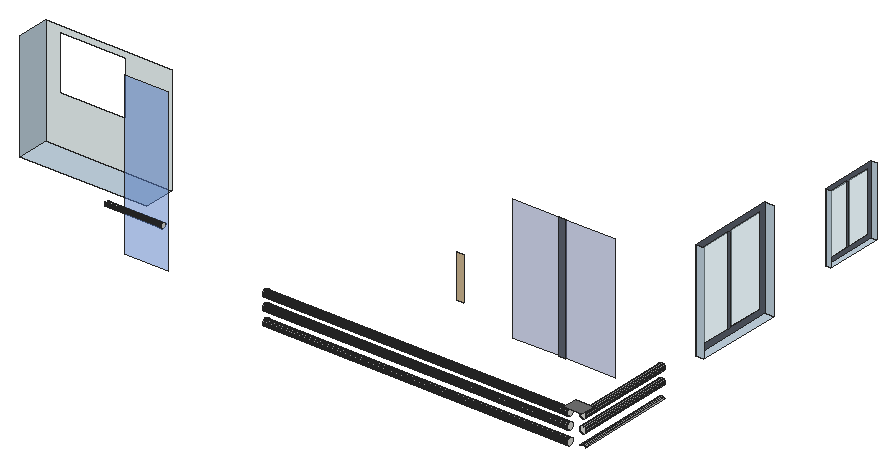
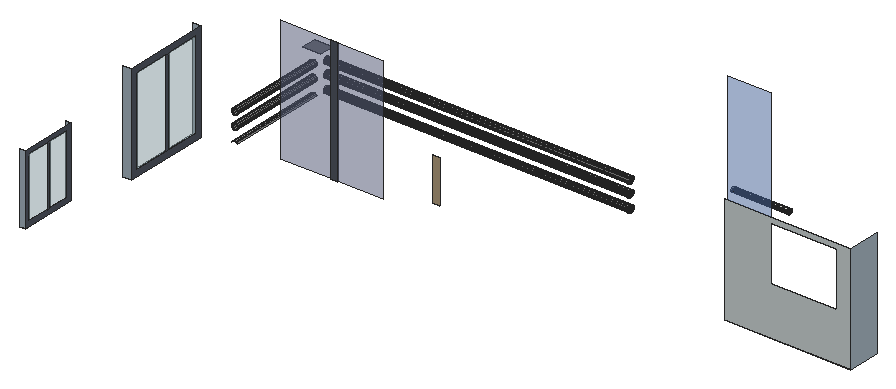
# SketchUp Ruby script. Lengths in inches.
U = 1.inch
M = Sketchup.active_model
def pt(a) = Geom::Point3d.new(a.map { |v| v * U })
def face(e, loops, mat)
  f = e.add_face(loops[0].map { |a| pt(a) })
  loops[1..].each { |l| e.add_face(l.map { |a| pt(a) }).erase! }
  f.material = f.back_material = mat if mat
  f
end
# faces: each face lists its corners as indices into pts; further lists are holes
def faces(e, pts, list, mat = nil) = list.each { |f| face(e, (f[0].is_a?(Array) ? f : [f]).map { |l| l.map { |i| pts[i] } }, mat) }
# xy, xz, yz: faces in a plane at the given z, y or x. An outline is a flat list of corners, or four numbers for a rectangle; further outlines are holes
def ring(l) = l.size == 4 ? [[l[0], l[1]], [l[2], l[1]], [l[2], l[3]], [l[0], l[3]]] : l.each_slice(2).to_a
def flat(e, list, mat, &to3) = list.each { |f| face(e, (f[0].is_a?(Array) ? f : [f]).map { |l| ring(l).map { |u, v| to3.(u, v) } }, mat) }
def xy(e, z, list, mat = nil) = flat(e, list, mat) { |x, y| [x, y, z] }
def xz(e, y, list, mat = nil) = flat(e, list, mat) { |x, z| [x, y, z] }
def yz(e, x, list, mat = nil) = flat(e, list, mat) { |y, z| [x, y, z] }
def lines(e, pts, list) = list.each { |a, b| e.add_line(pt(pts[a]), pt(pts[b])) }
# prism: a flat outline (further loops are holes) pulled along v
def prism(e, loops, v, mat = nil)
  f = face(e, loops, mat); d = Geom::Vector3d.new(v.map { |x| x * U })
  f.pushpull(f.normal.samedirection?(d) ? d.length : -d.length)
end
def box(e, o, s, mat = nil) = prism(e, [[o, [o[0] + s[0], o[1], o[2]], [o[0] + s[0], o[1] + s[1], o[2]], [o[0], o[1] + s[1], o[2]]]], [0, 0, s[2]], mat)
def at(x, y, z, deg = 0) = Geom::Transformation.translation(pt([x, y, z])) * Geom::Transformation.rotation(ORIGIN, Z_AXIS, deg.degrees)
def axes(o, x, y, z) = Geom::Transformation.new([*x, 0, *y, 0, *z, 0, *pt(o).to_a, 1])
def part(name) = M.definitions.add(name)
# library, detail: a bought-in or finely detailed component or shape, given as its bounding box
def library(name, o, s) = part(name).tap { |d| box(d.entities, o, s) }
def detail(e, o, s) = box(e.add_group.entities, o, s)
def put(e, d, t, mat = nil) = e.add_instance(d, t).tap { |i| i.material = mat if mat }
def group(e, t, mat = nil) = e.add_group.tap { |g| g.transformation = t; g.material = mat if mat }.entities
root = M.entities
M.materials.add("[Color M03]").color = [170, 170, 170]
M.materials.add("[Color M05]").color = [114, 114, 114]
M.materials.add("[Formica Beige]").color = [211, 187, 149]
M.materials.add("[Formica Laminate Dark]").color = [95, 101, 114]
M.materials.add("[Terrazzo Light Blue]1").color = [196, 214, 227]
M.materials.add("[Translucent Glass Blue]").color = [100, 149, 237]
M.materials["[Translucent Glass Blue]"].alpha = 0.5
M.materials.add("[Translucent Glass Safety]").color = [204, 235, 244]
M.materials["[Translucent Glass Safety]"].alpha = 0.5
M.materials.add("[Translucent Glass Sky Reflection]").color = [126, 138, 183]
M.materials["[Translucent Glass Sky Reflection]"].alpha = 0.52
M.materials.add("[White Subway Tile]").color = [243, 252, 253]
xy(root,1272.1,[[547.35,1118.14,1034.97,1239.01]],"[Terrazzo Light Blue]1")
xy(root,1302.22,[[2936.43,1390.76,2968.68,1726.13]],"[Terrazzo Light Blue]1")
xy(root,1339.25,[[2140.61,820.84,2143.62,821.24,2146.42,822.4,2148.83,824.25,2150.67,826.66,2151.84,829.46,2152.23,832.47,2151.84,835.48,2150.67,838.28,2148.83,840.69,2146.42,842.54,2143.62,843.7,2140.61,844.09,2137.6,843.7,2134.79,842.54,2132.39,840.69,2130.54,838.28,2129.38,835.48,2128.98,832.47,2129.38,829.46,2130.54,826.66,2132.39,824.25,2134.79,822.4,2137.6,821.24]])
xy(root,1348.11,[[2949.18,2002.64,2968.68,2223.02]],"[Terrazzo Light Blue]1")
xy(root,1369.75,[[2898.76,803.71,2968.68,859.31]],"[Color M05]")
xy(root,1433.45,[[1250.58,820.58,1251.73,820.73,1252.8,821.17,1253.72,821.88,1254.42,822.8,1254.87,823.87,1255.02,825.02,1254.87,826.17,1254.42,827.24,1253.72,828.15,1252.8,828.86,1251.73,829.3,1250.58,829.45,1249.43,829.3,1248.36,828.86,1247.44,828.15,1246.74,827.24,1246.29,826.17,1246.14,825.02,1246.29,823.87,1246.74,822.8,1247.44,821.88,1248.36,821.17,1249.43,820.73]])
xy(root,1436.77,[[1314.2,820.58,1315.35,820.73,1316.42,821.17,1317.34,821.88,1318.05,822.8,1318.49,823.87,1318.64,825.02,1318.49,826.17,1318.05,827.24,1317.34,828.15,1316.42,828.86,1315.35,829.3,1314.2,829.45,1313.06,829.3,1311.99,828.86,1311.07,828.15,1310.36,827.24,1309.92,826.17,1309.77,825.02,1309.92,823.87,1310.36,822.8,1311.07,821.88,1311.99,821.17,1313.06,820.73]])
xy(root,1437.08,[[1197.58,820.58,1198.73,820.73,1199.8,821.17,1200.72,821.88,1201.42,822.8,1201.87,823.87,1202.02,825.02,1201.87,826.17,1201.42,827.24,1200.72,828.15,1199.8,828.86,1198.73,829.3,1197.58,829.45,1196.43,829.3,1195.36,828.86,1194.44,828.15,1193.74,827.24,1193.29,826.17,1193.14,825.02,1193.29,823.87,1193.74,822.8,1194.44,821.88,1195.36,821.17,1196.43,820.73]])
xy(root,1437.8,[[1292.95,820.58,1294.1,820.73,1295.17,821.17,1296.09,821.88,1296.8,822.8,1297.24,823.87,1297.39,825.02,1297.24,826.17,1296.8,827.24,1296.09,828.15,1295.17,828.86,1294.1,829.3,1292.95,829.45,1291.81,829.3,1290.74,828.86,1289.82,828.15,1289.11,827.24,1288.67,826.17,1288.52,825.02,1288.67,823.87,1289.11,822.8,1289.82,821.88,1290.74,821.17,1291.81,820.73]])
xy(root,1440.11,[[1222.58,820.58,1223.73,820.73,1224.8,821.17,1225.72,821.88,1226.42,822.8,1226.87,823.87,1227.02,825.02,1226.87,826.17,1226.42,827.24,1225.72,828.15,1224.8,828.86,1223.73,829.3,1222.58,829.45,1221.43,829.3,1220.36,828.86,1219.44,828.15,1218.74,827.24,1218.29,826.17,1218.14,825.02,1218.29,823.87,1218.74,822.8,1219.44,821.88,1220.36,821.17,1221.43,820.73],[1271.08,820.58,1272.23,820.73,1273.3,821.17,1274.22,821.88,1274.92,822.8,1275.37,823.87,1275.52,825.02,1275.37,826.17,1274.92,827.24,1274.22,828.15,1273.3,828.86,1272.23,829.3,1271.08,829.45,1269.93,829.3,1268.86,828.86,1267.94,828.15,1267.24,827.24,1266.79,826.17,1266.64,825.02,1266.79,823.87,1267.24,822.8,1267.94,821.88,1268.86,821.17,1269.93,820.73]])
xy(root,1442.27,[[1131.58,820.58,1132.73,820.73,1133.8,821.17,1134.72,821.88,1135.42,822.8,1135.87,823.87,1136.02,825.02,1135.87,826.17,1135.42,827.24,1134.72,828.15,1133.8,828.86,1132.73,829.3,1131.58,829.45,1130.43,829.3,1129.36,828.86,1128.44,828.15,1127.74,827.24,1127.29,826.17,1127.14,825.02,1127.29,823.87,1127.74,822.8,1128.44,821.88,1129.36,821.17,1130.43,820.73],[1151.52,820.58,1152.67,820.73,1153.74,821.17,1154.65,821.88,1155.36,822.8,1155.8,823.87,1155.95,825.02,1155.8,826.17,1155.36,827.24,1154.65,828.15,1153.74,828.86,1152.67,829.3,1151.52,829.45,1150.37,829.3,1149.3,828.86,1148.38,828.15,1147.67,827.24,1147.23,826.17,1147.08,825.02,1147.23,823.87,1147.67,822.8,1148.38,821.88,1149.3,821.17,1150.37,820.73],[1173.58,820.58,1174.73,820.73,1175.8,821.17,1176.72,821.88,1177.42,822.8,1177.87,823.87,1178.02,825.02,1177.87,826.17,1177.42,827.24,1176.72,828.15,1175.8,828.86,1174.73,829.3,1173.58,829.45,1172.43,829.3,1171.36,828.86,1170.44,828.15,1169.74,827.24,1169.29,826.17,1169.14,825.02,1169.29,823.87,1169.74,822.8,1170.44,821.88,1171.36,821.17,1172.43,820.73]])
xz(root,859.31,[[2927.58,1264.46,2930.84,1264.89,2933.87,1266.15,2936.47,1268.14,2938.46,1270.75,2939.72,1273.77,2940.15,1277.03,2939.72,1280.28,2938.46,1283.31,2936.47,1285.91,2933.87,1287.91,2930.84,1289.16,2927.58,1289.59,2924.33,1289.16,2921.3,1287.91,2918.7,1285.91,2916.7,1283.31,2915.45,1280.28,2915.02,1277.03,2915.45,1273.77,2916.7,1270.75,2918.7,1268.14,2921.3,1266.15,2924.33,1264.89],[2927.58,1316.03,2930.84,1316.45,2933.87,1317.71,2936.47,1319.71,2938.46,1322.31,2939.72,1325.34,2940.15,1328.59,2939.72,1331.84,2938.46,1334.87,2936.47,1337.47,2933.87,1339.47,2930.84,1340.72,2927.58,1341.15,2924.33,1340.72,2921.3,1339.47,2918.7,1337.47,2916.7,1334.87,2915.45,1331.84,2915.02,1328.59,2915.45,1325.34,2916.7,1322.31,2918.7,1319.71,2921.3,1317.71,2924.33,1316.45]])
xz(root,884.27,[[1137.95,1242.25,1309.12,1865.04]],"[Translucent Glass Blue]")
xz(root,1239.01,[[2136.34,1281.23,2162.72,1446.98]],"[Formica Beige]")
xz(root,1239.01,[[2528.23,1224.02,2557.29,1706.3]],"[Formica Laminate Dark]")
xz(root,1239.01,[[2353.98,1224.02,2528.23,1706.3],[2557.29,1224.02,2749.1875,1706.3]],"[Translucent Glass Sky Reflection]")
xz(root,1239.01,[[[547.35,1272.1,1034.97,1690.66],[601.67,1457.66,858.23,1670.72]]],"[White Subway Tile]")
xz(root,1390.76,[[2936.43,1302.22,2968.68,1686.6]],"[Terrazzo Light Blue]1")
xz(root,1726.13,[[2936.43,1302.22,2968.68,1686.6]],"[Terrazzo Light Blue]1")
xz(root,2002.64,[[2949.18,1348.11,2968.68,1615.93]],"[Terrazzo Light Blue]1")
xz(root,2223.02,[[2949.18,1348.11,2968.68,1615.93]],"[Terrazzo Light Blue]1")
yz(root,547.35,[[1118.14,1272.1,1239.01,1690.66]],"[Terrazzo Light Blue]1")
yz(root,1334.04,[[826.07,1428.86,828.38,1429.16,830.54,1430.06,832.39,1431.48,833.8125,1433.33,834.7,1435.48,835.01,1437.8,834.7,1440.11,833.8125,1442.27,832.39,1444.12,830.54,1445.54,828.38,1446.43,826.07,1446.73,823.76,1446.43,821.6,1445.54,819.75,1444.12,818.33,1442.27,817.4375,1440.11,817.13,1437.8,817.4375,1435.48,818.33,1433.33,819.75,1431.48,821.6,1430.06,823.76,1429.16]])
yz(root,2898.76,[[834.19,1224.6,837.45,1225.03,840.48,1226.29,843.08,1228.28,845.07,1230.88,846.33,1233.91,846.76,1237.17,846.33,1240.42,845.07,1243.45,843.08,1246.05,840.48,1248.05,837.45,1249.3,834.19,1249.73,830.94,1249.3,827.91,1248.05,825.3125,1246.05,823.32,1243.45,822.06,1240.42,821.63,1237.17,822.06,1233.91,823.32,1230.88,825.3125,1228.28,827.91,1226.29,830.94,1225.03],[834.19,1277.73,837.45,1278.16,840.48,1279.41,843.08,1281.41,845.07,1284.01,846.33,1287.04,846.76,1290.29,846.33,1293.54,845.07,1296.57,843.08,1299.17,840.48,1301.17,837.45,1302.43,834.19,1302.85,830.94,1302.43,827.91,1301.17,825.3125,1299.17,823.32,1296.57,822.06,1293.54,821.63,1290.29,822.06,1287.04,823.32,1284.01,825.3125,1281.41,827.91,1279.41,830.94,1278.16],[834.19,1325.79,837.45,1326.22,840.48,1327.47,843.08,1329.47,845.07,1332.07,846.33,1335.1,846.76,1338.35,846.33,1341.6,845.07,1344.63,843.08,1347.24,840.48,1349.23,837.45,1350.49,834.19,1350.92,830.94,1350.49,827.91,1349.23,825.3125,1347.24,823.32,1344.63,822.06,1341.6,821.63,1338.35,822.06,1335.1,823.32,1332.07,825.3125,1329.47,827.91,1327.47,830.94,1326.22]])
yz(root,2936.43,[[[1390.76,1302.22,1726.13,1686.6],[1414.45,1325.92,1702.4375,1662.9]],[1545.625,1325.92,1562.55,1662.9]],"[Formica Laminate Dark]")
yz(root,2936.43,[[1414.45,1325.92,1545.625,1662.9],[1562.55,1325.92,1702.4375,1662.9]],"[Translucent Glass Safety]")
yz(root,2949.18,[[[2002.64,1348.11,2223.02,1615.93],[2020.78,1366.25,2204.875,1597.79]],[2104.71,1366.25,2115.27,1597.79]],"[Formica Laminate Dark]")
yz(root,2949.18,[[2020.78,1366.25,2104.71,1597.79],[2115.27,1366.25,2204.875,1597.79]],"[Translucent Glass Safety]")
p = [[2916.7,859.31,1219.62],[2918.7,859.31,1222.22],[2918.7,1239.01,1222.22],[2916.7,1239.01,1219.62],[2936.47,859.31,1222.22],[2938.46,859.31,1219.62],
  [2938.46,1239.01,1219.62],[2936.47,1239.01,1222.22],[2921.3,859.31,1224.22],[2921.3,1239.01,1224.22],[2933.87,859.31,1224.22],[2933.87,1239.01,1224.22],
  [2924.33,859.31,1225.47],[2924.33,1239.01,1225.47],[2930.84,859.31,1225.47],[2930.84,1239.01,1225.47],[2898.76,834.19,1224.6],[2898.76,830.94,1225.03],
  [1720.33,830.94,1225.03],[1720.33,834.19,1224.6],[2898.76,837.45,1225.03],[1720.33,837.45,1225.03],[2898.76,827.91,1226.29],[1720.33,827.91,1226.29],
  [2898.76,840.48,1226.29],[1720.33,840.48,1226.29],[2927.58,859.31,1225.9],[2927.58,1239.01,1225.9],[2898.76,825.3125,1228.28],[1720.33,825.3125,1228.28],
  [2898.76,843.08,1228.28],[1720.33,843.08,1228.28],[2898.76,823.32,1230.88],[1720.33,823.32,1230.88],[2898.76,845.07,1230.88],[1720.33,845.07,1230.88],
  [2898.76,822.06,1233.91],[1720.33,822.06,1233.91],[2898.76,846.33,1233.91],[1720.33,846.33,1233.91],[2898.76,821.63,1237.17],[1720.33,821.63,1237.17],
  [2898.76,846.76,1237.17],[1720.33,846.76,1237.17],[2898.76,822.06,1240.42],[1720.33,822.06,1240.42],[2898.76,846.33,1240.42],[1720.33,846.33,1240.42],
  [2898.76,823.32,1243.45],[1720.33,823.32,1243.45],[2898.76,845.07,1243.45],[1720.33,845.07,1243.45],[2898.76,825.3125,1246.05],[1720.33,825.3125,1246.05],
  [2898.76,843.08,1246.05],[1720.33,843.08,1246.05],[2898.76,827.91,1248.05],[1720.33,827.91,1248.05],[2898.76,840.48,1248.05],[1720.33,840.48,1248.05],
  [2898.76,830.94,1249.3],[1720.33,830.94,1249.3],[2898.76,837.45,1249.3],[1720.33,837.45,1249.3],[2898.76,834.19,1249.73],[1720.33,834.19,1249.73],
  [2927.58,859.31,1264.46],[2924.33,859.31,1264.89],[2924.33,1239.01,1264.89],[2927.58,1239.01,1264.46],[2930.84,859.31,1264.89],[2930.84,1239.01,1264.89],
  [2921.3,859.31,1266.15],[2921.3,1239.01,1266.15],[2933.87,859.31,1266.15],[2933.87,1239.01,1266.15],[2918.7,859.31,1268.14],[2918.7,1239.01,1268.14],
  [2936.47,859.31,1268.14],[2936.47,1239.01,1268.14],[2916.7,859.31,1270.75],[2916.7,1239.01,1270.75],[2938.46,859.31,1270.75],[2938.46,1239.01,1270.75],
  [2915.45,859.31,1273.77],[2915.45,1239.01,1273.77],[2939.72,859.31,1273.77],[2939.72,1239.01,1273.77],[2915.02,859.31,1277.03],[2915.02,1239.01,1277.03],
  [2940.15,859.31,1277.03],[2940.15,1239.01,1277.03],[2915.45,859.31,1280.28],[2915.45,1239.01,1280.28],[2939.72,859.31,1280.28],[2939.72,1239.01,1280.28],
  [2898.76,834.19,1277.73],[2898.76,830.94,1278.16],[1720.33,830.94,1278.16],[1720.33,834.19,1277.73],[2898.76,837.45,1278.16],[1720.33,837.45,1278.16],
  [2898.76,827.91,1279.41],[1720.33,827.91,1279.41],[2898.76,840.48,1279.41],[1720.33,840.48,1279.41],[2898.76,825.3125,1281.41],[1720.33,825.3125,1281.41],
  [2898.76,843.08,1281.41],[1720.33,843.08,1281.41],[2916.7,859.31,1283.31],[2916.7,1239.01,1283.31],[2938.46,859.31,1283.31],[2938.46,1239.01,1283.31],
  [2898.76,823.32,1284.01],[1720.33,823.32,1284.01],[2898.76,845.07,1284.01],[1720.33,845.07,1284.01],[2918.7,859.31,1285.91],[2918.7,1239.01,1285.91],
  [2936.47,859.31,1285.91],[2936.47,1239.01,1285.91],[2898.76,822.06,1287.04],[1720.33,822.06,1287.04],[2898.76,846.33,1287.04],[1720.33,846.33,1287.04],
  [2921.3,859.31,1287.91],[2921.3,1239.01,1287.91],[2933.87,859.31,1287.91],[2933.87,1239.01,1287.91],[2898.76,821.63,1290.29],[1720.33,821.63,1290.29],
  [2898.76,846.76,1290.29],[1720.33,846.76,1290.29],[2924.33,859.31,1289.16],[2924.33,1239.01,1289.16],[2930.84,859.31,1289.16],[2930.84,1239.01,1289.16],
  [2927.58,859.31,1289.59],[2927.58,1239.01,1289.59],[2898.76,822.06,1293.54],[1720.33,822.06,1293.54],[2898.76,846.33,1293.54],[1720.33,846.33,1293.54],
  [2898.76,823.32,1296.57],[1720.33,823.32,1296.57],[2898.76,845.07,1296.57],[1720.33,845.07,1296.57],[2898.76,825.3125,1299.17],[1720.33,825.3125,1299.17],
  [2898.76,843.08,1299.17],[1720.33,843.08,1299.17],[2898.76,827.91,1301.17],[1720.33,827.91,1301.17],[2898.76,840.48,1301.17],[1720.33,840.48,1301.17],
  [2898.76,830.94,1302.43],[1720.33,830.94,1302.43],[2898.76,837.45,1302.43],[1720.33,837.45,1302.43],[2898.76,834.19,1302.85],[1720.33,834.19,1302.85],
  [2927.58,859.31,1316.03],[2924.33,859.31,1316.45],[2924.33,1239.01,1316.45],[2927.58,1239.01,1316.03],[2930.84,859.31,1316.45],[2930.84,1239.01,1316.45],
  [2921.3,859.31,1317.71],[2921.3,1239.01,1317.71],[2933.87,859.31,1317.71],[2933.87,1239.01,1317.71],[2918.7,859.31,1319.71],[2918.7,1239.01,1319.71],
  [2936.47,859.31,1319.71],[2936.47,1239.01,1319.71],[2916.7,859.31,1322.31],[2916.7,1239.01,1322.31],[2938.46,859.31,1322.31],[2938.46,1239.01,1322.31],
  [2915.45,859.31,1325.34],[2915.45,1239.01,1325.34],[2939.72,859.31,1325.34],[2939.72,1239.01,1325.34],[2915.02,859.31,1328.59],[2915.02,1239.01,1328.59],
  [2940.15,859.31,1328.59],[2940.15,1239.01,1328.59],[2898.76,834.19,1325.79],[2898.76,830.94,1326.22],[1720.33,830.94,1326.22],[1720.33,834.19,1325.79],
  [2898.76,837.45,1326.22],[1720.33,837.45,1326.22],[2898.76,827.91,1327.47],[1720.33,827.91,1327.47],[2898.76,840.48,1327.47],[1720.33,840.48,1327.47],
  [2898.76,825.3125,1329.47],[1720.33,825.3125,1329.47],[2898.76,843.08,1329.47],[1720.33,843.08,1329.47],[2915.45,859.31,1331.84],[2915.45,1239.01,1331.84],
  [2939.72,859.31,1331.84],[2939.72,1239.01,1331.84],[2898.76,823.32,1332.07],[1720.33,823.32,1332.07],[2898.76,845.07,1332.07],[1720.33,845.07,1332.07],
  [2916.7,859.31,1334.87],[2916.7,1239.01,1334.87],[2938.46,859.31,1334.87],[2938.46,1239.01,1334.87],[2898.76,822.06,1335.1],[1720.33,822.06,1335.1],
  [2898.76,846.33,1335.1],[1720.33,846.33,1335.1],[2918.7,859.31,1337.47],[2918.7,1239.01,1337.47],[2936.47,859.31,1337.47],[2936.47,1239.01,1337.47],
  [2898.76,821.63,1338.35],[1720.33,821.63,1338.35],[2898.76,846.76,1338.35],[1720.33,846.76,1338.35],[2921.3,859.31,1339.47],[2921.3,1239.01,1339.47],
  [2933.87,859.31,1339.47],[2933.87,1239.01,1339.47],[2898.76,822.06,1341.6],[1720.33,822.06,1341.6],[2898.76,846.33,1341.6],[1720.33,846.33,1341.6],
  [2924.33,859.31,1340.72],[2924.33,1239.01,1340.72],[2930.84,859.31,1340.72],[2930.84,1239.01,1340.72],[2927.58,859.31,1341.15],[2927.58,1239.01,1341.15],
  [2898.76,823.32,1344.63],[1720.33,823.32,1344.63],[2898.76,845.07,1344.63],[1720.33,845.07,1344.63],[2898.76,825.3125,1347.24],[1720.33,825.3125,1347.24],
  [2898.76,843.08,1347.24],[1720.33,843.08,1347.24],[2898.76,827.91,1349.23],[1720.33,827.91,1349.23],[2898.76,840.48,1349.23],[1720.33,840.48,1349.23],
  [2898.76,830.94,1350.49],[1720.33,830.94,1350.49],[2898.76,837.45,1350.49],[1720.33,837.45,1350.49],[2898.76,834.19,1350.92],[1720.33,834.19,1350.92],
  [1334.04,826.07,1428.86],[1334.04,823.76,1429.16],[1113.04,823.76,1429.16],[1113.04,826.07,1428.86],[1334.04,828.38,1429.16],[1113.04,828.38,1429.16],
  [1334.04,821.6,1430.06],[1113.04,821.6,1430.06],[1334.04,830.54,1430.06],[1113.04,830.54,1430.06],[1334.04,819.75,1431.48],[1113.04,819.75,1431.48],
  [1334.04,832.39,1431.48],[1113.04,832.39,1431.48],[1334.04,818.33,1433.33],[1113.04,818.33,1433.33],[1334.04,833.8125,1433.33],[1113.04,833.8125,1433.33],
  [1334.04,817.4375,1435.48],[1113.04,817.4375,1435.48],[1334.04,834.7,1435.48],[1113.04,834.7,1435.48],[1334.04,817.13,1437.8],[1113.04,817.13,1437.8],
  [1334.04,835.01,1437.8],[1113.04,835.01,1437.8],[1334.04,817.4375,1440.11],[1113.04,817.4375,1440.11],[1334.04,834.7,1440.11],[1113.04,834.7,1440.11],
  [1334.04,818.33,1442.27],[1113.04,818.33,1442.27],[1334.04,833.8125,1442.27],[1113.04,833.8125,1442.27],[1334.04,819.75,1444.12],[1113.04,819.75,1444.12],
  [1334.04,832.39,1444.12],[1113.04,832.39,1444.12]]
faces(root,p,[[0,1,2,3],[4,5,6,7],[1,8,9,2],[10,4,7,11],[8,12,13,9],[14,10,11,15],[16,17,18,19],[20,16,19,21],
  [17,22,23,18],[24,20,21,25],[12,26,27,13],[26,14,15,27],[22,28,29,23],[30,24,25,31],[28,32,33,29],[34,30,31,35],
  [32,36,37,33],[38,34,35,39],[36,40,41,37],[42,38,39,43],[40,44,45,41],[46,42,43,47],[44,48,49,45],[50,46,47,51],
  [48,52,53,49],[54,50,51,55],[52,56,57,53],[58,54,55,59],[56,60,61,57],[62,58,59,63],[60,64,65,61],[64,62,63,65],
  [66,67,68,69],[70,66,69,71],[67,72,73,68],[74,70,71,75],[72,76,77,73],[78,74,75,79],[76,80,81,77],[82,78,79,83],
  [80,84,85,81],[86,82,83,87],[84,88,89,85],[90,86,87,91],[88,92,93,89],[94,90,91,95],[96,97,98,99],[100,96,99,101],
  [97,102,103,98],[104,100,101,105],[102,106,107,103],[108,104,105,109],[92,110,111,93],[112,94,95,113],[106,114,115,107],[116,108,109,117],
  [110,118,119,111],[120,112,113,121],[114,122,123,115],[124,116,117,125],[118,126,127,119],[128,120,121,129],[122,130,131,123],[132,124,125,133],
  [126,134,135,127],[136,128,129,137],[134,138,139,135],[138,136,137,139],[130,140,141,131],[142,132,133,143],[140,144,145,141],[146,142,143,147],
  [144,148,149,145],[150,146,147,151],[148,152,153,149],[154,150,151,155],[152,156,157,153],[158,154,155,159],[156,160,161,157],[160,158,159,161],
  [162,163,164,165],[166,162,165,167],[163,168,169,164],[170,166,167,171],[168,172,173,169],[174,170,171,175],[172,176,177,173],[178,174,175,179],
  [176,180,181,177],[182,178,179,183],[180,184,185,181],[186,182,183,187],[188,189,190,191],[192,188,191,193],[189,194,195,190],[196,192,193,197],
  [194,198,199,195],[200,196,197,201],[184,202,203,185],[204,186,187,205],[198,206,207,199],[208,200,201,209],[202,210,211,203],[212,204,205,213],
  [206,214,215,207],[216,208,209,217],[210,218,219,211],[220,212,213,221],[214,222,223,215],[224,216,217,225],[218,226,227,219],[228,220,221,229],
  [222,230,231,223],[232,224,225,233],[226,234,235,227],[236,228,229,237],[234,238,239,235],[238,236,237,239],[230,240,241,231],[242,232,233,243],
  [240,244,245,241],[246,242,243,247],[244,248,249,245],[250,246,247,251],[248,252,253,249],[254,250,251,255],[252,256,257,253],[256,254,255,257],
  [258,259,260,261],[262,258,261,263],[259,264,265,260],[266,262,263,267],[264,268,269,265],[270,266,267,271],[268,272,273,269],[274,270,271,275],
  [272,276,277,273],[278,274,275,279],[276,280,281,277],[282,278,279,283],[280,284,285,281],[286,282,283,287],[284,288,289,285],[290,286,287,291],
  [288,292,293,289],[294,290,291,295]],"[Color M03]")
